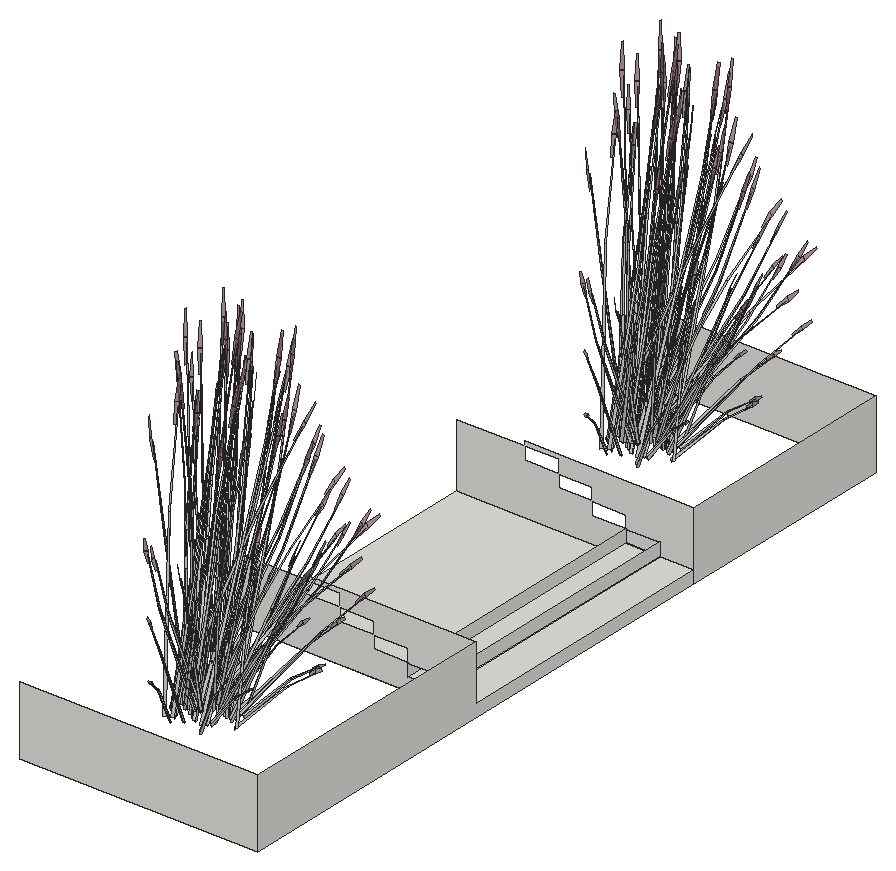
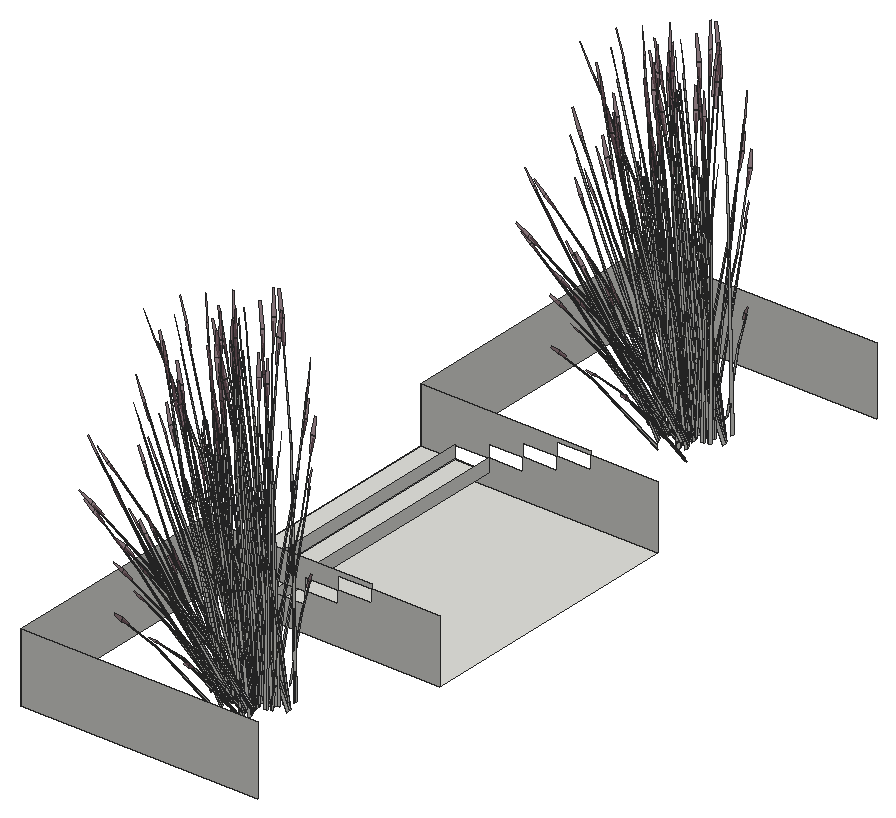
# SketchUp Ruby script. Lengths in inches.
U = 1.inch
M = Sketchup.active_model
def pt(a) = Geom::Point3d.new(a.map { |v| v * U })
def face(e, loops, mat)
  f = e.add_face(loops[0].map { |a| pt(a) })
  loops[1..].each { |l| e.add_face(l.map { |a| pt(a) }).erase! }
  f.material = f.back_material = mat if mat
  f
end
# faces: each face lists its corners as indices into pts; further lists are holes
def faces(e, pts, list, mat = nil) = list.each { |f| face(e, (f[0].is_a?(Array) ? f : [f]).map { |l| l.map { |i| pts[i] } }, mat) }
# xy, xz, yz: faces in a plane at the given z, y or x. An outline is a flat list of corners, or four numbers for a rectangle; further outlines are holes
def ring(l) = l.size == 4 ? [[l[0], l[1]], [l[2], l[1]], [l[2], l[3]], [l[0], l[3]]] : l.each_slice(2).to_a
def flat(e, list, mat, &to3) = list.each { |f| face(e, (f[0].is_a?(Array) ? f : [f]).map { |l| ring(l).map { |u, v| to3.(u, v) } }, mat) }
def xy(e, z, list, mat = nil) = flat(e, list, mat) { |x, y| [x, y, z] }
def xz(e, y, list, mat = nil) = flat(e, list, mat) { |x, z| [x, y, z] }
def yz(e, x, list, mat = nil) = flat(e, list, mat) { |y, z| [x, y, z] }
def lines(e, pts, list) = list.each { |a, b| e.add_line(pt(pts[a]), pt(pts[b])) }
# prism: a flat outline (further loops are holes) pulled along v
def prism(e, loops, v, mat = nil)
  f = face(e, loops, mat); d = Geom::Vector3d.new(v.map { |x| x * U })
  f.pushpull(f.normal.samedirection?(d) ? d.length : -d.length)
end
def box(e, o, s, mat = nil) = prism(e, [[o, [o[0] + s[0], o[1], o[2]], [o[0] + s[0], o[1] + s[1], o[2]], [o[0], o[1] + s[1], o[2]]]], [0, 0, s[2]], mat)
def at(x, y, z, deg = 0) = Geom::Transformation.translation(pt([x, y, z])) * Geom::Transformation.rotation(ORIGIN, Z_AXIS, deg.degrees)
def axes(o, x, y, z) = Geom::Transformation.new([*x, 0, *y, 0, *z, 0, *pt(o).to_a, 1])
def part(name) = M.definitions.add(name)
# library, detail: a bought-in or finely detailed component or shape, given as its bounding box
def library(name, o, s) = part(name).tap { |d| box(d.entities, o, s) }
def detail(e, o, s) = box(e.add_group.entities, o, s)
def put(e, d, t, mat = nil) = e.add_instance(d, t).tap { |i| i.material = mat if mat }
def group(e, t, mat = nil) = e.add_group.tap { |g| g.transformation = t; g.material = mat if mat }.entities
root = M.entities
M.materials.add("LightPink_Translucent").color = [144, 107, 117]
M.materials["LightPink_Translucent"].alpha = 0.75
c1 = part("blade")
p = [[2.15,0.21,22],[0,0.17,0],[0.09,0.45,0],[2.18,0.31,22],[2.29,0.31,22],[0.38,0.45,0],
  [2.48,0.24,33],[2.49,0.24,33],[2.48,0.22,33]]
faces(c1.entities,p,[[0,1,2,3],[4,5,2,3],[6,3,4,7],[8,0,3,6]])
c2 = part("seeds")
p = [[0.3,-0.1,1.38],[-0.01,-0.03,1.59],[-0.01,-0.03,0.03],[0.14,-0.07,-0.07],[0.29,-0.03,3],[0.15,0.01,3.11]]
faces(c2.entities,p,[[0,1,2,3],[1,0,4,5]],"LightPink_Translucent")
c3 = part("blade with seeds")
put(c3.entities,c1,at(0,0,0))
put(c3.entities,c2,axes([2.4,0.25,30.99],[1.5799,-0.05474,1.17369],[-0.12525,1.92788,0.29478],[-0.07173,-0.02425,1.56792]))
xy(root,0,[[480,48,515.75,96]])
xy(root,2.25,[[509.78,48,515.75,96],[515.75,48,521.72,96]])
xz(root,0,[[480,0,521.72,12]])
xz(root,48,[[[480,0,480,11.26,491.86,11.26,491.86,9.01,497.83,9.01,497.83,11.26,491.86,11.26,491.86,12,521.72,12,521.72,2.25,515.75,2.25,515.75,0],[497.83,6.76,503.8,9.01],[503.8,4.51,509.78,6.76],[509.78,2.25,515.75,4.51]]])
xz(root,96,[[[480,0,515.75,0,515.75,2.25,521.72,2.25,521.72,12,491.86,12,491.86,11.26,497.83,11.26,497.83,9.01,491.86,9.01,491.86,11.26,480,11.26],[509.78,2.25,515.75,4.51],[503.8,4.51,509.78,6.76],[497.83,6.76,503.8,9.01]],[509.78,2.25,515.75,4.51]])
xz(root,136.05,[[480,0,521.72,12]])
yz(root,509.78,[[48,2.25,96,4.51]])
yz(root,515.75,[[48,0,96,2.25],[48,2.25,96,4.51]])
yz(root,521.72,[[0,0,96,0,96,2.25,48,2.25,48,12,0,12],[96,0,136.05,12]])
put(root,c3,axes([491.18,22.75,2.36],[0.53281,1.15808,0.45755],[-1.52239,0.4027,0.17955],[0.01861,-0.2128,1.58856]))
put(root,c3,axes([490.9375,118.6,2.21],[0.59459,-0.93321,-0.44739],[1.23546,0.44912,0.21531],[0,-0.21512,1.43643]))
put(root,c3,axes([490.9375,22.6,2.21],[0.59459,-0.93321,-0.44739],[1.23546,0.44912,0.21531],[0,-0.21512,1.43643]))
put(root,c3,axes([492.46,121.61,2.2],[-0.39985,-0.89288,0],[1.1418,-0.31268,0],[0,0,1.54371]))
put(root,c3,axes([492.46,25.61,2.2],[-0.39985,-0.89288,0],[1.1418,-0.31268,0],[0,0,1.54371]))
put(root,c3,axes([491.01,123.49,1.49],[0.19833,-0.05635,1.76342],[1.19302,0.31018,-0.26939],[0.03489,0.3496,0.30037]))
put(root,c3,axes([491.01,27.49,1.49],[0.19833,-0.05635,1.76342],[1.19302,0.31018,-0.26939],[0.03489,0.3496,0.30037]))
put(root,c3,axes([491.27,123.81,4.53],[-0.36946,0.79643,-0.35414],[-1.07787,-0.23229,0.4572],[0.09883,0.32066,0.87481]))
put(root,c3,axes([491.27,27.81,4.53],[-0.36946,0.79643,-0.35414],[-1.07787,-0.23229,0.4572],[0.09883,0.32066,0.87481]))
put(root,c3,axes([494.07,119.85,2.21],[-0.59459,0.93321,-0.44739],[-1.23546,-0.44912,0.21531],[0,0.21512,1.43643]))
put(root,c3,axes([494.07,23.85,2.21],[-0.59459,0.93321,-0.44739],[-1.23546,-0.44912,0.21531],[0,0.21512,1.43643]))
put(root,c3,axes([496.42,119.28,2.47],[-0.96285,-0.75439,0.17642],[0.97031,-0.7317,0.35086],[-0.10634,0.15406,1.60407]))
put(root,c3,axes([496.42,23.28,2.47],[-0.96285,-0.75439,0.17642],[0.97031,-0.7317,0.35086],[-0.10634,0.15406,1.60407]))
put(root,c3,axes([493.1,118.85,2.21],[0,-1.19833,0],[1.53239,0,0],[0,0,1.79456]))
put(root,c3,axes([493.1,22.85,2.21],[0,-1.19833,0],[1.53239,0,0],[0,0,1.79456]))
put(root,c3,axes([491.67,119.0625,2.43],[1.3808,0.50196,0.24065],[-0.66454,1.04299,0.50002],[0,-0.24043,1.60543]))
put(root,c3,axes([491.67,23.0625,2.43],[1.3808,0.50196,0.24065],[-0.66454,1.04299,0.50002],[0,-0.24043,1.60543]))
put(root,c3,axes([493.87,119.32,2.29],[0,1.19774,-0.05637],[-1.53239,0,0],[0,0.03764,1.79368]))
put(root,c3,axes([493.87,23.32,2.29],[0,1.19774,-0.05637],[-1.53239,0,0],[0,0.03764,1.79368]))
put(root,c3,axes([491.23,118.37,2.72],[-1.33077,0.06393,0.44739],[-0.12035,-1.06125,-0.21531],[0.23824,-0.10756,1.43643]))
put(root,c3,axes([491.23,22.37,2.72],[-1.33077,0.06393,0.44739],[-0.12035,-1.06125,-0.21531],[0.23824,-0.10756,1.43643]))
put(root,c3,axes([490.61,116.54,2.47],[-0.35402,1.02926,0.17642],[-1.29548,-0.29127,0.35086],[0.22379,-0.00501,1.60407]))
put(root,c3,axes([490.61,20.54,2.47],[-0.35402,1.02926,0.17642],[-1.29548,-0.29127,0.35086],[0.22379,-0.00501,1.60407]))
put(root,c3,axes([493.14,121.64,2.29],[0.53281,1.18979,-0.06012],[-1.52239,0.41691,0],[0.01861,0.04155,1.72173]))
put(root,c3,axes([493.14,25.64,2.29],[0.53281,1.18979,-0.06012],[-1.52239,0.41691,0],[0.01861,0.04155,1.72173]))
put(root,c3,axes([489.97,115.27,2.375],[-0.7662,-1.03778,0],[1.28187,-0.57875,-0.51607],[0.29196,-0.13181,1.63711]))
put(root,c3,axes([489.97,19.27,2.375],[-0.7662,-1.03778,0],[1.28187,-0.57875,-0.51607],[0.29196,-0.13181,1.63711]))
put(root,c3,axes([491.38,123.09,4.98],[0.5849,0.8421,-0.71045],[-1.20401,0.4693,0.08574],[0.13677,0.40688,1.00501]))
put(root,c3,axes([491.38,27.09,4.98],[0.5849,0.8421,-0.71045],[-1.20401,0.4693,0.08574],[0.13677,0.40688,1.00501]))
put(root,c3,axes([497.54,120.08,2.2],[-1.53164,-0.00828,-0.04976],[0,-1.1575,0.49943],[-0.04813,0.2635,1.58352]))
put(root,c3,axes([497.54,24.08,2.2],[-1.53164,-0.00828,-0.04976],[0,-1.1575,0.49943],[-0.04813,0.2635,1.58352]))
put(root,c3,axes([494.53,116.6,2.47],[-1.31687,0.27488,0.17642],[-0.32517,-1.02297,0.35086],[0.11745,0.14905,1.60407]))
put(root,c3,axes([494.53,20.6,2.47],[-1.31687,0.27488,0.17642],[-0.32517,-1.02297,0.35086],[0.11745,0.14905,1.60407]))
put(root,c3,axes([493.18,112.77,2.77],[0.15721,0.60392,1.1486],[-0.87211,-0.33448,0.84392],[0.09385,-0.30923,0.25299]))
put(root,c3,axes([493.18,16.77,2.77],[0.15721,0.60392,1.1486],[-0.87211,-0.33448,0.84392],[0.09385,-0.30923,0.25299]))
put(root,c3,axes([492.37,118.09,2.36],[-1.01611,0.93987,0.45755],[-1.20717,-0.82966,0.17955],[0.24496,-0.0938,1.58856]))
put(root,c3,axes([492.37,22.09,2.36],[-1.01611,0.93987,0.45755],[-1.20717,-0.82966,0.17955],[0.24496,-0.0938,1.58856]))
put(root,c3,axes([494.11,119.57,2.21],[0.85545,0.66896,0],[-0.85545,0.66896,0],[0,0,1.69266]))
put(root,c3,axes([494.11,23.57,2.21],[0.85545,0.66896,0],[-0.85545,0.66896,0],[0,0,1.69266]))
put(root,c3,axes([494.1,118.79,2.72],[0.59459,-0.93321,0.44739],[1.23546,0.44912,-0.21531],[0,0.21512,1.43643]))
put(root,c3,axes([494.1,22.79,2.72],[0.59459,-0.93321,0.44739],[1.23546,0.44912,-0.21531],[0,0.21512,1.43643]))
put(root,c3,axes([493.58,122.03,2.2],[1.23546,0.46496,0],[-0.59459,0.96613,0],[0,0,1.74954]))
put(root,c3,axes([493.58,26.03,2.2],[1.23546,0.46496,0],[-0.59459,0.96613,0],[0,0,1.74954]))
put(root,c3,axes([491.82,123.26,4.68],[1.20468,0.25962,-0.51099],[-0.41292,0.89013,-0.3958],[0.11046,0.35838,0.97773]))
put(root,c3,axes([491.82,27.26,4.68],[1.20468,0.25962,-0.51099],[-0.41292,0.89013,-0.3958],[0.11046,0.35838,0.97773]))
put(root,c3,axes([493.7,118.57,2.38],[-1.54892,-0.2182,0.49198],[0.31522,-1.23236,0.19306],[0.22636,0.119,1.70813]))
put(root,c3,axes([493.7,22.57,2.38],[-1.54892,-0.2182,0.49198],[0.31522,-1.23236,0.19306],[0.22636,0.119,1.70813]))
put(root,c3,axes([497.22,120.25,2.03],[-0.85545,0.64616,-0.30978],[-0.85545,-0.64616,0.30978],[0,0.20813,1.38974]))
put(root,c3,axes([497.22,24.25,2.03],[-0.85545,0.64616,-0.30978],[-0.85545,-0.64616,0.30978],[0,0.20813,1.38974]))
put(root,c3,axes([494.77,120.13,2.09],[0.44936,0.94823,-0.69212],[-1.29441,0.3415,-0.18165],[0.04967,0.32109,1.52773]))
put(root,c3,axes([494.77,24.13,2.09],[0.44936,0.94823,-0.69212],[-1.29441,0.3415,-0.18165],[0.04967,0.32109,1.52773]))
put(root,c3,axes([494.14,119.11,2.21],[1.37109,0,0],[0,1.07219,0],[0,0,1.78407]))
put(root,c3,axes([494.14,23.11,2.21],[1.37109,0,0],[0,1.07219,0],[0,0,1.78407]))
put(root,c3,axes([492.82,117.93,2.72],[-0.73619,-0.86927,0.44739],[1.11511,-0.61213,-0.21531],[0.23824,0.10756,1.43643]))
put(root,c3,axes([492.82,21.93,2.72],[-0.73619,-0.86927,0.44739],[1.11511,-0.61213,-0.21531],[0.23824,0.10756,1.43643]))
put(root,c3,axes([491.48,118.14,2.67],[-0.1428,-1.18174,-0.29095],[1.48733,-0.07145,-0.50002],[0.26191,-0.15741,1.59708]))
put(root,c3,axes([491.48,22.14,2.67],[-0.1428,-1.18174,-0.29095],[1.48733,-0.07145,-0.50002],[0.26191,-0.15741,1.59708]))
put(root,c3,axes([494.61,119,2.62],[1.1418,-0.30203,0.1448],[0.39985,0.86246,-0.41347],[0,0.18981,1.26744]))
put(root,c3,axes([494.61,23,2.62],[1.1418,-0.30203,0.1448],[0.39985,0.86246,-0.41347],[0,0.18981,1.26744]))
put(root,c3,axes([495.04,115.67,4.68],[-0.87728,-0.69587,-0.51099],[0.92674,-0.60943,-0.3958],[0.13348,-0.35356,0.97773]))
put(root,c3,axes([495.04,19.67,4.68],[-0.87728,-0.69587,-0.51099],[0.92674,-0.60943,-0.3958],[0.13348,-0.35356,0.97773]))
put(root,c3,axes([494.22,119.07,2.67],[1.38012,0.49416,-0.29095],[-0.66454,1.04299,-0.50002],[0.04337,0.25608,1.59708]))
put(root,c3,axes([494.22,23.07,2.67],[1.38012,0.49416,-0.29095],[-0.66454,1.04299,-0.50002],[0.04337,0.25608,1.59708]))
put(root,c3,axes([491.28,115.52,2.03],[1.14332,0.25625,-0.30978],[-0.28787,0.90242,0.30978],[0.23049,-0.10406,1.38974]))
put(root,c3,axes([491.28,19.52,2.03],[1.14332,0.25625,-0.30978],[-0.28787,0.90242,0.30978],[0.23049,-0.10406,1.38974]))
put(root,c3,axes([494.46,114.43,2.59],[-0.34835,0.20963,1.43002],[-1.04325,-0.36691,-0.30754],[0.19338,-0.4563,0.61141]))
put(root,c3,axes([494.46,18.43,2.59],[-0.34835,0.20963,1.43002],[-1.04325,-0.36691,-0.30754],[0.19338,-0.4563,0.61141]))
put(root,c3,axes([497.22,119.31,2.48],[0,-1.03566,0.49651],[1.37109,0,0],[0,0.23588,1.57504]))
put(root,c3,axes([497.22,23.31,2.48],[0,-1.03566,0.49651],[1.37109,0,0],[0,0.23588,1.57504]))
put(root,c3,axes([497.81,120.27,2.02],[0,1.03566,-0.49651],[-1.37109,0,0],[0,0.23588,1.57504]))
put(root,c3,axes([497.81,24.27,2.02],[0,1.03566,-0.49651],[-1.37109,0,0],[0,0.23588,1.57504]))
put(root,c3,axes([491.01,115.11,2.02],[1.14694,-0.51783,-0.49651],[0.68554,0.92854,0],[0.26122,-0.11794,1.57504]))
put(root,c3,axes([491.01,19.11,2.02],[1.14694,-0.51783,-0.49651],[0.68554,0.92854,0],[0.26122,-0.11794,1.57504]))
put(root,c3,axes([492.5,121.43,3.875],[-0.28013,-0.33252,1.71376],[1.29445,-0.27994,0.13857],[0.29256,0.52202,0.73262]))
put(root,c3,axes([492.5,25.43,3.875],[-0.28013,-0.33252,1.71376],[1.29445,-0.27994,0.13857],[0.29256,0.52202,0.73262]))
put(root,c3,axes([493.3125,117.6875,2.62],[0.23642,-0.92427,0.1448],[1.15506,0.16044,-0.41347],[0.21021,0.09491,1.26744]))
put(root,c3,axes([493.3125,21.6875,2.62],[0.23642,-0.92427,0.1448],[1.15506,0.16044,-0.41347],[0.21021,0.09491,1.26744]))
put(root,c3,axes([494.96,116.08,2.48],[-1.14694,-0.51783,0.49651],[0.68554,-0.92854,0],[0.26122,0.11794,1.57504]))
put(root,c3,axes([494.96,20.08,2.48],[-1.14694,-0.51783,0.49651],[0.68554,-0.92854,0],[0.26122,0.11794,1.57504]))
put(root,c3,axes([495.3125,115.99,4.98],[0.03189,-0.95798,-0.71045],[1.34277,0.06434,0.08574],[0.14171,-0.40585,1.00501]))
put(root,c3,axes([495.3125,19.99,4.98],[0.03189,-0.95798,-0.71045],[1.34277,0.06434,0.08574],[0.14171,-0.40585,1.00501]))
put(root,c3,axes([493.96,121.48,2.18],[1.2866,-0.3514,-0.19198],[0.45209,1.01223,0.00008],[0.14202,-0.03884,1.73897]))
put(root,c3,axes([493.96,25.48,2.18],[1.2866,-0.3514,-0.19198],[0.45209,1.01223,0.00008],[0.14202,-0.03884,1.73897]))
put(root,c3,axes([493.98,118.48,2.21],[0.73619,0.86927,-0.44739],[-1.11511,0.61213,0.21531],[0.23824,0.10756,1.43643]))
put(root,c3,axes([493.98,22.48,2.21],[0.73619,0.86927,-0.44739],[-1.11511,0.61213,0.21531],[0.23824,0.10756,1.43643]))
put(root,c3,axes([495.87,115.41,4.53],[0.82919,-0.54528,-0.35414],[0.78493,0.62262,0.4572],[0.11943,-0.31634,0.87481]))
put(root,c3,axes([495.87,19.41,4.53],[0.82919,-0.54528,-0.35414],[0.78493,0.62262,0.4572],[0.11943,-0.31634,0.87481]))
put(root,c3,axes([496.0625,122.42,2.77],[-0.69001,-0.29779,1.1486],[0.89096,-0.30257,0.84392],[0.24031,0.2563,0.25299]))
put(root,c3,axes([496.0625,26.42,2.77],[-0.69001,-0.29779,1.1486],[0.89096,-0.30257,0.84392],[0.24031,0.2563,0.25299]))
put(root,c3,axes([493.61,122.1,2.59],[0.02163,-0.34331,1.43002],[1.03345,-0.38348,-0.30754],[0.31903,0.4109,0.61141]))
put(root,c3,axes([493.61,26.1,2.59],[0.02163,-0.34331,1.43002],[1.03345,-0.38348,-0.30754],[0.31903,0.4109,0.61141]))
put(root,c3,axes([492.375,117.24,2.06],[0.82544,-0.77843,-0.62353],[1.0254,0.70586,-0.16365],[0.33076,-0.19418,1.37633]))
put(root,c3,axes([492.375,21.24,2.06],[0.82544,-0.77843,-0.62353],[1.0254,0.70586,-0.16365],[0.33076,-0.19418,1.37633]))
put(root,c3,axes([496,116.55,2.03],[0.28787,0.90242,-0.30978],[-1.14332,0.25625,0.30978],[0.23049,0.10406,1.38974]))
put(root,c3,axes([496,20.55,2.03],[0.28787,0.90242,-0.30978],[-1.14332,0.25625,0.30978],[0.23049,0.10406,1.38974]))
put(root,c3,axes([498.15,119.49,2.375],[1.53239,0,0],[0,1.1575,-0.51607],[0,0.26363,1.63711]))
put(root,c3,axes([498.15,23.49,2.375],[1.53239,0,0],[0,1.1575,-0.51607],[0,0.26363,1.63711]))
put(root,c3,axes([493.2,117.99,2.67],[1.23732,-0.68758,-0.29095],[0.8228,0.97154,-0.50002],[0.30528,0.09867,1.59708]))
put(root,c3,axes([493.2,21.99,2.67],[1.23732,-0.68758,-0.29095],[0.8228,0.97154,-0.50002],[0.30528,0.09867,1.59708]))
put(root,c3,axes([496.17,123.78,2.67],[-0.78586,-0.03248,1.0506],[0.51898,-0.68985,0.58006],[0.31045,0.24509,0.8241]))
put(root,c3,axes([496.17,27.78,2.67],[-0.78586,-0.03248,1.0506],[0.51898,-0.68985,0.58006],[0.31045,0.24509,0.8241]))
put(root,c3,axes([493.8,115.5,3.875],[-0.22818,0.35597,1.71376],[-0.95725,-0.73667,0.13857],[0.43183,-0.45914,0.73262]))
put(root,c3,axes([493.8,19.5,3.875],[-0.22818,0.35597,1.71376],[-0.95725,-0.73667,0.13857],[0.43183,-0.45914,0.73262]))
put(root,c3,axes([490.07,117.375,1.59],[-1.20625,0.41464,1.28929],[-0.38394,-1.1897,0.50096],[0.74071,0.01979,1.46642]))
put(root,c3,axes([490.07,21.375,1.59],[-1.20625,0.41464,1.28929],[-0.38394,-1.1897,0.50096],[0.74071,0.01979,1.46642]))
put(root,c3,axes([494.51,122.83,4.68],[1.20928,-0.24619,-0.51099],[0.21154,0.93233,-0.3958],[0.32481,0.26718,0.97773]))
put(root,c3,axes([494.51,26.83,4.68],[1.20928,-0.24619,-0.51099],[0.21154,0.93233,-0.3958],[0.32481,0.26718,0.97773]))
put(root,c3,axes([495.62,115.53,2.375],[0.7662,-1.03778,0],[1.28187,0.57875,-0.51607],[0.29196,0.13181,1.63711]))
put(root,c3,axes([495.62,19.53,2.375],[0.7662,-1.03778,0],[1.28187,0.57875,-0.51607],[0.29196,0.13181,1.63711]))
put(root,c3,axes([496.9,115.08,1.49],[-0.18342,-0.08159,1.76342],[-0.47115,-0.9115,-0.26939],[0.31784,-0.24736,0.30037]))
put(root,c3,axes([496.9,19.08,1.49],[-0.18342,-0.08159,1.76342],[-0.47115,-0.9115,-0.26939],[0.31784,-0.24736,0.30037]))
put(root,c3,axes([496.31,116.16,2.02],[1.14694,0.51783,-0.49651],[-0.68554,0.92854,0],[0.26122,0.11794,1.57504]))
put(root,c3,axes([496.31,20.16,2.02],[1.14694,0.51783,-0.49651],[-0.68554,0.92854,0],[0.26122,0.11794,1.57504]))
put(root,c3,axes([496.26,123.53,1.49],[0.08928,-0.14952,1.76342],[1.12407,-0.44035,-0.26939],[0.34078,0.22791,0.30037]))
put(root,c3,axes([496.26,27.53,1.49],[0.08928,-0.14952,1.76342],[1.12407,-0.44035,-0.26939],[0.34078,0.22791,0.30037]))
put(root,c3,axes([496.86,117.27,4.68],[-0.31482,-0.94565,-0.51099],[1.19224,-0.16542,-0.3958],[0.34166,-0.254,0.97773]))
put(root,c3,axes([496.86,21.27,4.68],[-0.31482,-0.94565,-0.51099],[1.19224,-0.16542,-0.3958],[0.34166,-0.254,0.97773]))
put(root,c3,axes([498.96,122.15,3.93],[-0.23455,-0.87059,-0.03492],[1.10861,-0.20015,-0.15832],[0.23151,0.05519,0.52218]))
put(root,c3,axes([498.96,26.15,3.93],[-0.23455,-0.87059,-0.03492],[1.10861,-0.20015,-0.15832],[0.23151,0.05519,0.52218]))
put(root,c3,axes([494.64,118.14,2.06],[1.27479,0.1698,-0.62353],[-0.26901,1.04736,-0.16365],[0.38043,0.12691,1.37633]))
put(root,c3,axes([494.64,22.14,2.06],[1.27479,0.1698,-0.62353],[-0.26901,1.04736,-0.16365],[0.38043,0.12691,1.37633]))
put(root,c3,axes([500.07,118.76,2.26],[-0.75977,-0.66224,-0.06488],[0.83212,-0.6068,-0.29416],[0.23578,-0.04272,0.97024]))
put(root,c3,axes([500.07,22.76,2.26],[-0.75977,-0.66224,-0.06488],[0.83212,-0.6068,-0.29416],[0.23578,-0.04272,0.97024]))
put(root,c3,axes([498.33,115.39,2.77],[-0.40819,0.5272,1.1486],[-0.35086,-0.70831,0.84392],[0.33713,-0.17749,0.25299]))
put(root,c3,axes([498.33,19.39,2.77],[-0.40819,0.5272,1.1486],[-0.35086,-0.70831,0.84392],[0.33713,-0.17749,0.25299]))
put(root,c3,axes([494.38,120.39,3.875],[-0.45521,-0.17844,1.71376],[0.94204,-0.74856,0.13857],[0.58713,0.33769,0.73262]))
put(root,c3,axes([494.38,24.39,3.875],[-0.45521,-0.17844,1.71376],[0.94204,-0.74856,0.13857],[0.58713,0.33769,0.73262]))
put(root,c3,axes([497.74,117.37,4.53],[1.06674,-0.14801,-0.35414],[0.28168,0.84611,0.4572],[0.30569,-0.22726,0.87481]))
put(root,c3,axes([497.74,21.37,4.53],[1.06674,-0.14801,-0.35414],[0.28168,0.84611,0.4572],[0.30569,-0.22726,0.87481]))
put(root,c3,axes([496.89,117.65,4.98],[0.64013,-0.81717,-0.71045],[1.12174,0.58074,0.08574],[0.38221,-0.29607,1.00501]))
put(root,c3,axes([496.89,21.65,4.98],[0.64013,-0.81717,-0.71045],[1.12174,0.58074,0.08574],[0.38221,-0.29607,1.00501]))
put(root,c3,axes([496.88,122.05,4.53],[0.69728,0.64842,-0.35414],[-0.79619,0.61382,0.4572],[0.40453,0.09339,0.87481]))
put(root,c3,axes([496.88,26.05,4.53],[0.69728,0.64842,-0.35414],[-0.79619,0.61382,0.4572],[0.40453,0.09339,0.87481]))
put(root,c3,axes([497.42,119.37,4.68],[0.332,-0.94205,-0.51099],[1.13828,0.3229,-0.3958],[0.45829,-0.08638,0.97773]))
put(root,c3,axes([497.42,23.37,4.68],[0.332,-0.94205,-0.51099],[1.13828,0.3229,-0.3958],[0.45829,-0.08638,0.97773]))
put(root,c3,axes([500.27,119.97,2.77],[-0.75718,0.17097,1.1486],[0.35641,-0.70661,0.84392],[0.40168,0.04835,0.25299]))
put(root,c3,axes([500.27,23.97,2.77],[-0.75718,0.17097,1.1486],[0.35641,-0.70661,0.84392],[0.40168,0.04835,0.25299]))
put(root,c3,axes([497.82,116.9,2.59],[-0.4378,-0.03068,1.43002],[-0.44851,-0.8229,-0.30754],[0.53783,-0.23279,0.61141]))
put(root,c3,axes([497.82,20.9,2.59],[-0.4378,-0.03068,1.43002],[-0.44851,-0.8229,-0.30754],[0.53783,-0.23279,0.61141]))
put(root,c3,axes([498.11,119.8,4.53],[1.01846,0.28891,-0.35414],[-0.29705,0.84289,0.4572],[0.41005,-0.07729,0.87481]))
put(root,c3,axes([498.11,23.8,4.53],[1.01846,0.28891,-0.35414],[-0.29705,0.84289,0.4572],[0.41005,-0.07729,0.87481]))
put(root,c3,axes([496.15,121.62,4.98],[1.22504,0.02494,-0.71045],[-0.08228,1.05005,0.08574],[0.51899,0.11081,1.00501]))
put(root,c3,axes([496.15,25.62,4.98],[1.22504,0.02494,-0.71045],[-0.08228,1.05005,0.08574],[0.51899,0.11081,1.00501]))
put(root,c3,axes([498.63,119.64,1.98],[-0.7893,0.12429,1.41583],[-0.12563,-0.9893,0.08104],[0.55282,-0.14974,0.80566]))
put(root,c3,axes([498.63,23.64,1.98],[-0.7893,0.12429,1.41583],[-0.12563,-0.9893,0.08104],[0.55282,-0.14974,0.80566]))
put(root,c3,axes([499.49,118.99,1.49],[-0.06405,-0.15723,1.76342],[0.44421,-0.91974,-0.26939],[0.4481,-0.01323,0.30037]))
put(root,c3,axes([499.49,22.99,1.49],[-0.06405,-0.15723,1.76342],[0.44421,-0.91974,-0.26939],[0.4481,-0.01323,0.30037]))
put(root,c3,axes([495.34,118.76,3.875],[-0.50831,0.02346,1.71376],[0.33721,-1.01661,0.13857],[0.72439,0.06288,0.73262]))
put(root,c3,axes([495.34,22.76,3.875],[-0.50831,0.02346,1.71376],[0.33721,-1.01661,0.13857],[0.72439,0.06288,0.73262]))
put(root,c3,axes([497.2,119.71,4.98],[1.07686,-0.45739,-0.71045],[0.60013,0.94154,0.08574],[0.52031,-0.10696,1.00501]))
put(root,c3,axes([497.2,23.71,4.98],[1.07686,-0.45739,-0.71045],[0.60013,0.94154,0.08574],[0.52031,-0.10696,1.00501]))
put(root,c3,axes([498.86,121.11,2.59],[-0.29514,-0.25472,1.43002],[0.38401,-0.84262,-0.30754],[0.59714,0.11414,0.61141]))
put(root,c3,axes([498.86,25.11,2.59],[-0.29514,-0.25472,1.43002],[0.38401,-0.84262,-0.30754],[0.59714,0.11414,0.61141]))
